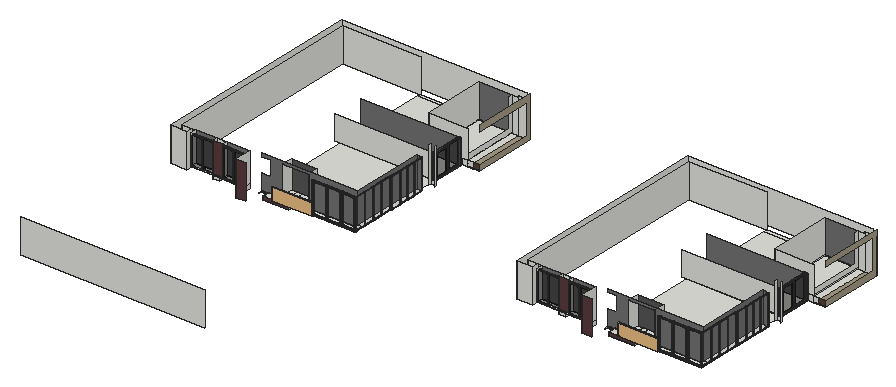
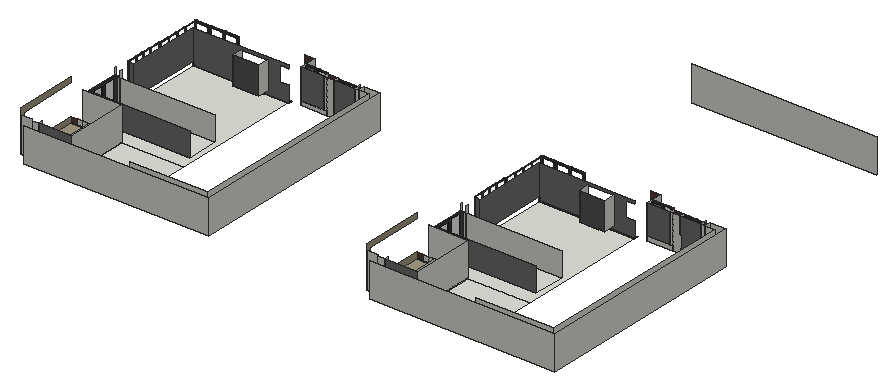
# SketchUp Ruby script. Lengths in inches.
U = 1.inch
M = Sketchup.active_model
def pt(a) = Geom::Point3d.new(a.map { |v| v * U })
def face(e, loops, mat)
  f = e.add_face(loops[0].map { |a| pt(a) })
  loops[1..].each { |l| e.add_face(l.map { |a| pt(a) }).erase! }
  f.material = f.back_material = mat if mat
  f
end
# faces: each face lists its corners as indices into pts; further lists are holes
def faces(e, pts, list, mat = nil) = list.each { |f| face(e, (f[0].is_a?(Array) ? f : [f]).map { |l| l.map { |i| pts[i] } }, mat) }
# xy, xz, yz: faces in a plane at the given z, y or x. An outline is a flat list of corners, or four numbers for a rectangle; further outlines are holes
def ring(l) = l.size == 4 ? [[l[0], l[1]], [l[2], l[1]], [l[2], l[3]], [l[0], l[3]]] : l.each_slice(2).to_a
def flat(e, list, mat, &to3) = list.each { |f| face(e, (f[0].is_a?(Array) ? f : [f]).map { |l| ring(l).map { |u, v| to3.(u, v) } }, mat) }
def xy(e, z, list, mat = nil) = flat(e, list, mat) { |x, y| [x, y, z] }
def xz(e, y, list, mat = nil) = flat(e, list, mat) { |x, z| [x, y, z] }
def yz(e, x, list, mat = nil) = flat(e, list, mat) { |y, z| [x, y, z] }
def lines(e, pts, list) = list.each { |a, b| e.add_line(pt(pts[a]), pt(pts[b])) }
# prism: a flat outline (further loops are holes) pulled along v
def prism(e, loops, v, mat = nil)
  f = face(e, loops, mat); d = Geom::Vector3d.new(v.map { |x| x * U })
  f.pushpull(f.normal.samedirection?(d) ? d.length : -d.length)
end
def box(e, o, s, mat = nil) = prism(e, [[o, [o[0] + s[0], o[1], o[2]], [o[0] + s[0], o[1] + s[1], o[2]], [o[0], o[1] + s[1], o[2]]]], [0, 0, s[2]], mat)
def at(x, y, z, deg = 0) = Geom::Transformation.translation(pt([x, y, z])) * Geom::Transformation.rotation(ORIGIN, Z_AXIS, deg.degrees)
def axes(o, x, y, z) = Geom::Transformation.new([*x, 0, *y, 0, *z, 0, *pt(o).to_a, 1])
def part(name) = M.definitions.add(name)
# library, detail: a bought-in or finely detailed component or shape, given as its bounding box
def library(name, o, s) = part(name).tap { |d| box(d.entities, o, s) }
def detail(e, o, s) = box(e.add_group.entities, o, s)
def put(e, d, t, mat = nil) = e.add_instance(d, t).tap { |i| i.material = mat if mat }
def group(e, t, mat = nil) = e.add_group.tap { |g| g.transformation = t; g.material = mat if mat }.entities
root = M.entities
M.materials.add("Glass_Tinted_Gray").color = [0, 0, 0]
M.materials["Glass_Tinted_Gray"].alpha = 0.125
M.materials.add("Glazing").color = [128, 128, 128]
M.materials["Glazing"].alpha = 0.05
M.materials.add("Powdercoating").color = [41, 44, 40]
M.materials.add("Wine2").color = [0, 0, 0]
M.materials["Wine2"].alpha = 0
M.materials.add("[0130_Gainsboro]").color = [39, 45, 50]
M.materials.add("[0135_DarkGray]").color = [81, 81, 81]
M.materials.add("[Color M05]").color = [114, 114, 114]
M.materials.add("[Color M06]").color = [86, 86, 86]
M.materials.add("[Concrete Tile]").color = [165, 155, 133]
M.materials.add("[Granite Brown]").color = [89, 59, 61]
M.materials.add("[Granite Brown]1").color = [89, 63, 50]
M.materials.add("[Mirror 02]").color = [229, 229, 229]
M.materials.add("[Terrazzo Light Blue]").color = [196, 214, 227]
c1 = library("Glass Railing",[0,0,0],[139.5,4.76,42])
c2 = part("Framed glazing panel")
xy(c2.entities,0,[[0,-0.98,43.07,0],[0,0,43.07,1.4]],"[0130_Gainsboro]")
xy(c2.entities,0.3,[[0.3,-1.43,42.77,-0.98]],"[0130_Gainsboro]")
xy(c2.entities,2.95,[[2.95,-1.43,40.12,-0.63],[2.95,-0.63,40.12,0],[2.95,0,40.12,0.64],[2.95,0.64,40.12,1.4]],"[0130_Gainsboro]")
xy(c2.entities,3.54,[[3.54,-0.63,39.53,0],[3.54,0,39.53,0.64]],"[0130_Gainsboro]")
xy(c2.entities,111.8125,[[3.54,-0.63,39.53,0],[3.54,0,39.53,0.64]],"[0130_Gainsboro]")
xy(c2.entities,112.4,[[2.95,-1.43,40.12,-0.63],[2.95,-0.63,40.12,0],[2.95,0,40.12,0.64],[2.95,0.64,40.12,1.4]],"[0130_Gainsboro]")
xy(c2.entities,115.05,[[0.3,-1.43,42.77,-0.98]],"[0130_Gainsboro]")
xy(c2.entities,115.35,[[0,-0.98,43.07,0],[0,0,43.07,1.4]],"[0130_Gainsboro]")
xz(c2.entities,-1.43,[[[0.3,0.3,42.77,115.05],[2.95,2.95,40.12,112.4]]],"[0130_Gainsboro]")
xz(c2.entities,-0.98,[[[0,0,43.07,115.35],[0.3,0.3,42.77,115.05]]],"[0130_Gainsboro]")
xz(c2.entities,-0.63,[[[2.95,2.95,40.12,112.4],[3.54,3.54,39.53,111.8125]]],"[0130_Gainsboro]")
xz(c2.entities,0,[[3.54,3.54,39.53,111.8125]],"Wine2")
xz(c2.entities,0,[[[0,0,43.07,115.35],[2.95,2.95,40.12,112.4]],[[2.95,2.95,40.12,112.4],[3.54,3.54,39.53,111.8125]]],"[0130_Gainsboro]")
xz(c2.entities,0.64,[[[2.95,2.95,40.12,112.4],[3.54,3.54,39.53,111.8125]]],"[0130_Gainsboro]")
xz(c2.entities,1.4,[[[0,0,43.07,115.35],[2.95,2.95,40.12,112.4]]],"[0130_Gainsboro]")
yz(c2.entities,0,[[-0.98,0,0,115.35],[0,0,1.4,115.35]],"[0130_Gainsboro]")
yz(c2.entities,0.3,[[-1.43,0.3,-0.98,115.05]],"[0130_Gainsboro]")
yz(c2.entities,2.95,[[-1.43,2.95,-0.63,112.4],[-0.63,2.95,0,112.4],[0,2.95,0.64,112.4],[0.64,2.95,1.4,112.4]],"[0130_Gainsboro]")
yz(c2.entities,3.54,[[-0.63,3.54,0,111.8125],[0,3.54,0.64,111.8125]],"[0130_Gainsboro]")
yz(c2.entities,39.53,[[-0.63,3.54,0,111.8125],[0,3.54,0.64,111.8125]],"[0130_Gainsboro]")
yz(c2.entities,40.12,[[-1.43,2.95,-0.63,112.4],[-0.63,2.95,0,112.4],[0,2.95,0.64,112.4],[0.64,2.95,1.4,112.4]],"[0130_Gainsboro]")
yz(c2.entities,42.77,[[-1.43,0.3,-0.98,115.05]],"[0130_Gainsboro]")
yz(c2.entities,43.07,[[-0.98,0,0,115.35],[0,0,1.4,115.35]],"[0130_Gainsboro]")
c3 = part("Glazed panel assembly")
put(c3.entities,c2,axes([90.57,1.43,0],[1.05148,0,0],[0,1,0],[0,0,1]))
put(c3.entities,c2,axes([0,1.43,0],[1.05148,0,0],[0,1,0],[0,0,1]))
put(c3.entities,c2,axes([45.29,1.43,0],[1.05148,0,0],[0,1,0],[0,0,1]))
c4 = part("PENTEK_RP Fineline 50S_Sliding_DoorCase_E1")
box(c4.entities,[0,0,0],[1.51,3.66,99.27],"[0135_DarkGray]")
c5 = part("PENTEK_RP Fineline 50S_SlidingDooe_Case_E2")
box(c5.entities,[0,0,0],[96.25,3.66,1.51],"[0135_DarkGray]")
c6 = part("pentek_RP Fineline 50S_SlidingDoor_Case")
put(c6.entities,c4,at(97.76,0,0))
put(c6.entities,c5,at(1.51,0,0))
put(c6.entities,c4,at(0,0,0))
put(c6.entities,c5,at(1.51,0,97.76))
c7 = part("PENTEK_RP Fineline 50S_SlidingDoor_GlazingBead_2")
box(c7.entities,[0,0,0],[0.56,0.59,94.39],"[0135_DarkGray]")
c8 = part("PENTEK_RP Fineline 50S_SlidingDoor_Glass")
box(c8.entities,[0,0,0],[46.58,0.16,94.39],"Glass_Tinted_Gray")
c9 = part("PENTEK_RP Fineline 50S_SlidingDoor_GlazingBead")
box(c9.entities,[0,0,0],[45.47,0.59,0.56],"[0135_DarkGray]")
c10 = part("PENTEK_RP Fineline 50S_SlidingDoor_Leaf_E1")
xy(c10.entities,0,[[0,0,0.93,1.97],[0.93,1.57,1.49,1.97]],"[0135_DarkGray]")
xy(c10.entities,96.25,[[0,0,0.93,0,0.93,1.57,1.49,1.57,1.49,1.97,0,1.97]],"[0135_DarkGray]")
xz(c10.entities,0,[[0,0,0.93,96.25]],"[0135_DarkGray]")
xz(c10.entities,1.57,[[0.93,0,1.49,95.32],[0.93,95.32,1.49,96.25]],"[0135_DarkGray]")
xz(c10.entities,1.97,[[0,0,1.49,96.25]],"[0135_DarkGray]")
yz(c10.entities,0,[[0,0,1.97,96.25]],"[0135_DarkGray]")
yz(c10.entities,0.93,[[0,0,1.57,0.93],[0,0.93,1.57,95.32],[0,95.32,1.57,96.25]],"[0135_DarkGray]")
yz(c10.entities,1.49,[[1.57,0,1.97,95.32],[1.57,95.32,1.97,96.25]],"[0135_DarkGray]")
c11 = part("PENTEK_RP Fineline 50S_SlidingDoor_Leaf_E2")
xy(c11.entities,0,[[0,0,0,1.57,0.56,1.57,0.56,1.97,46.02,1.97,46.02,1.57,46.58,1.57,46.58,0]],"[0135_DarkGray]")
xy(c11.entities,0.93,[[0,0,46.58,1.57]],"[0135_DarkGray]")
xy(c11.entities,1.49,[[0.56,1.57,46.02,1.97]],"[0135_DarkGray]")
xz(c11.entities,0,[[0,0,46.58,0.93]],"[0135_DarkGray]")
xz(c11.entities,1.57,[[0,0,0.56,0.93],[46.02,0,46.58,0.93],[0.56,0.93,46.02,1.49]],"[0135_DarkGray]")
xz(c11.entities,1.97,[[0.56,0,46.02,1.49]],"[0135_DarkGray]")
yz(c11.entities,0,[[0,0,1.57,0.93]],"[0135_DarkGray]")
yz(c11.entities,0.56,[[1.57,0,1.97,0.93],[1.57,0.93,1.97,1.49]],"[0135_DarkGray]")
yz(c11.entities,46.02,[[1.57,0,1.97,0.93],[1.57,0.93,1.97,1.49]],"[0135_DarkGray]")
yz(c11.entities,46.58,[[0,0,1.57,0.93]],"[0135_DarkGray]")
c12 = part("PENTEK_RP Fineline S_SlidingDoor_Leaf1")
put(c12.entities,c7,at(0.93,0,0.93))
put(c12.entities,c7,at(46.96,0,0.93))
put(c12.entities,c8,at(1.49,1.42,0.93))
put(c12.entities,c9,at(1.49,0,0.93))
put(c12.entities,c8,at(1.49,0.59,0.93),"[Terrazzo Light Blue]")
put(c12.entities,c10,at(0,0,0))
put(c12.entities,c10,axes([48.44,0,0],[-1,0,0],[0,1,0],[0,0,1]))
put(c12.entities,c11,axes([0.93,0,96.25],[1,0,0],[0,1,0],[0,0,-1]))
put(c12.entities,c11,at(0.93,0,0))
put(c12.entities,c9,at(1.49,0,94.77))
c13 = part("PENTEK_RP Fineline 50S_SlidingDoor_Leaf2")
put(c13.entities,c8,at(1.49,1.42,0.93))
put(c13.entities,c9,at(1.49,0,94.77))
put(c13.entities,c7,at(46.96,0,0.93))
put(c13.entities,c8,at(1.49,0.59,0.93),"[Mirror 02]")
put(c13.entities,c7,at(0.93,0,0.93))
put(c13.entities,c10,at(0,0,0))
put(c13.entities,c10,axes([48.44,0,0],[-1,0,0],[0,1,0],[0,0,1]))
put(c13.entities,c9,at(1.49,0,0.93))
put(c13.entities,c11,axes([0.93,0,96.25],[1,0,0],[0,1,0],[0,0,-1]))
put(c13.entities,c11,at(0.93,0,0))
c14 = part("PENTEK - Slimmest Steel Sliding Door / Window\#1")
put(c14.entities,c6,at(0,-1.88,-0.09))
put(c14.entities,c12,at(1.51,-2.27,1.42))
put(c14.entities,c13,at(49.32,-0.3,1.42))
c15 = part("Group\#15")
xy(c15.entities,0,[[0,-55.94,0.71,45.94]])
xy(c15.entities,0.2,[[0,-55.94,0.47,45.94],[0.47,45.94,0.71,46.42]])
xy(c15.entities,2.36,[[0.47,-55.94,0.71,46.42]])
xz(c15.entities,-55.94,[[0,0,0.71,0,0.71,2.36,0.47,2.36,0.47,0.2,0,0.2]])
xz(c15.entities,45.94,[[0,0,0.71,0.2]])
xz(c15.entities,46.42,[[0.47,0.2,0.71,2.36]])
yz(c15.entities,0,[[-55.94,0,45.94,0.2]])
yz(c15.entities,0.47,[[-55.94,0.2,46.42,2.36]])
yz(c15.entities,0.71,[[-55.94,0,45.94,0,45.94,0.2,46.42,0.2,46.42,2.36,-55.94,2.36]])
c16 = part("Group\#7")
xy(c16.entities,0,[[0,-59.09,0.71,45.94]])
xy(c16.entities,0.2,[[0,-59.09,0.47,45.94],[0.47,45.94,0.71,46.42]])
xy(c16.entities,2.36,[[0.47,-59.09,0.71,46.42]])
xz(c16.entities,-59.09,[[0,0,0.71,0,0.71,2.36,0.47,2.36,0.47,0.2,0,0.2]])
xz(c16.entities,45.94,[[0,0,0.71,0.2]])
xz(c16.entities,46.42,[[0.47,0.2,0.71,2.36]])
yz(c16.entities,0,[[-59.09,0,45.94,0.2]])
yz(c16.entities,0.47,[[-59.09,0.2,46.42,2.36]])
yz(c16.entities,0.71,[[-59.09,0,45.94,0,45.94,0.2,46.42,0.2,46.42,2.36,-59.09,2.36]])
c17 = part("Group\#16")
prism(c17.entities,[[[0.47,-56.18,0.2],[0,-56.18,0.2],[0,-56.18,0],[0.71,-56.18,0],[0.71,-56.18,2.36],[0.47,-56.18,2.36]]],[0,28.68,0])
c18 = part("Group\#10")
box(c18.entities,[-0.73,0,0],[27.99,0.55,102.05])
c19 = part("Group\#18")
xy(c19.entities,0,[[0.47,-56.18,0.47,-55.47,0,-55.47,0,-28.21,1.18,-28.21,1.18,-56.18]])
xy(c19.entities,0.2,[[0.71,-56.18,1.18,-28.21],[0,-55.47,0.47,-28.21],[0.47,-28.21,0.71,-27.74]])
xy(c19.entities,2.36,[[0.47,-56.18,0.71,-27.74]])
xz(c19.entities,-56.18,[[0.47,0,1.18,0,1.18,0.2,0.71,0.2,0.71,2.36,0.47,2.36]])
xz(c19.entities,-55.47,[[0,0,0.47,0.2]])
xz(c19.entities,-28.21,[[0,0,1.18,0.2]])
xz(c19.entities,-27.74,[[0.47,0.2,0.71,2.36]])
yz(c19.entities,0,[[-55.47,0,-28.21,0.2]])
yz(c19.entities,0.47,[[-56.18,0,-55.47,0.2],[-56.18,0.2,-27.74,2.36]])
yz(c19.entities,0.71,[[-56.18,0.2,-27.74,2.36]])
yz(c19.entities,1.18,[[-56.18,0,-28.21,0.2]])
c20 = part("Group\#34")
xy(c20.entities,0,[[-20.45,0,7.76,1.22]])
xy(c20.entities,0.06,[[-20.39,0.06,7.7,1.22]])
xy(c20.entities,0.47,[[-19.98,0,7.28,0.06]])
xy(c20.entities,101.89,[[-19.98,0,7.28,0.06]])
xy(c20.entities,102.3,[[-20.39,0.06,7.7,1.22]])
xy(c20.entities,102.36,[[-20.45,0,7.76,1.22]])
xz(c20.entities,0,[[[-20.45,0,7.76,102.36],[-19.98,0.47,7.28,101.89]]])
xz(c20.entities,0.06,[[[-20.39,0.06,7.7,102.3],[-19.98,0.47,7.28,101.89]]])
xz(c20.entities,1.22,[[[-20.45,0,7.76,102.36],[-20.39,0.06,7.7,102.3]]])
yz(c20.entities,-20.45,[[0,0,1.22,102.36]])
yz(c20.entities,-20.39,[[0.06,0.06,1.22,102.3]])
yz(c20.entities,-19.98,[[0,0.47,0.06,101.89]])
yz(c20.entities,7.28,[[0,0.47,0.06,101.89]])
yz(c20.entities,7.7,[[0.06,0.06,1.22,102.3]])
yz(c20.entities,7.76,[[0,0,1.22,102.36]])
c21 = part("Group\#6")
put(c21.entities,c15,axes([27.97,0,7.875],[1,0,0],[0,0,-1],[0,1,0]),"Powdercoating")
put(c21.entities,c16,axes([0.71,0,6.8],[-1,0,0],[0,0,-0.97687],[0,1,0]),"Powdercoating")
put(c21.entities,c17,axes([-27.5,0,-38.07],[0,0,-1],[-1,0,0],[0,1,0]),"Powdercoating")
put(c21.entities,c18,at(1.12,0.35,-38.39),"Glazing")
put(c21.entities,c19,axes([-27.5,0,63.35],[0,0,1],[-1,0,0],[0,1,0]),"Powdercoating")
put(c21.entities,c20,at(20.6875,1.0625,-38.54),"Powdercoating")
c22 = part("Sliding door assembly")
put(c22.entities,c21,at(-1.18,4.5,38.86))
g1 = group(c22.entities,at(84.74,4.5,38.86))
put(g1,c15,axes([-27.97,0,7.875],[-1,0,0],[0,0,-1],[0,1,0]),"Powdercoating")
put(g1,c16,axes([-0.71,0,6.8],[1,0,0],[0,0,-0.97687],[0,1,0]),"Powdercoating")
put(g1,c17,axes([27.5,0,-38.07],[0,0,-1],[1,0,0],[0,1,0]),"Powdercoating")
put(g1,c18,axes([-1.12,0.35,-38.39],[-1,0,0],[0,1,0],[0,0,1]),"Glazing")
put(g1,c19,axes([27.5,0,63.35],[0,0,1],[1,0,0],[0,1,0]),"Powdercoating")
put(g1,c20,axes([-20.6875,1.0625,-38.54],[-1,0,0],[0,1,0],[0,0,1]),"Powdercoating")
g2 = group(c22.entities,at(56.0625,4.5,38.86))
put(g2,c15,axes([-27.97,0,7.875],[-1,0,0],[0,0,-1],[0,1,0]),"Powdercoating")
put(g2,c17,axes([27.5,0,-38.07],[0,0,-1],[1,0,0],[0,1,0]),"Powdercoating")
put(g2,c18,axes([-1.12,0.35,-38.39],[-1,0,0],[0,1,0],[0,0,1]),"Glazing")
put(g2,c19,axes([27.5,0,63.35],[0,0,1],[1,0,0],[0,1,0]),"Powdercoating")
put(g2,c20,axes([-20.6875,1.0625,-38.54],[-1,0,0],[0,1,0],[0,0,1]),"Powdercoating")
g3 = group(g2,at(-0.71,0,6.8),"Powdercoating")
xy(g3,-45.34,[[0.47,0.2,0.71,2.36]])
xy(g3,-44.88,[[0,0,0.71,0.2]])
xy(g3,57.73,[[0,0,0.71,0,0.71,2.36,0.47,2.36,0.47,0.2,0,0.2]])
xz(g3,0,[[0,-44.88,0.71,57.73]])
xz(g3,0.2,[[0.47,-45.34,0.71,-44.88],[0,-44.88,0.47,57.73]])
xz(g3,2.36,[[0.47,-45.34,0.71,57.73]])
yz(g3,0,[[0,-44.88,0.2,57.73]])
yz(g3,0.47,[[0.2,-45.34,2.36,57.73]])
yz(g3,0.71,[[0.2,-45.34,2.36,-45.34,2.36,57.73,0,57.73,0,-44.88,0.2,-44.88]])
put(c22.entities,c21,axes([-33.94,4.5,38.86],[1.14218,0,0],[0,1,0],[0,0,1]))
c23 = part("sliding door")
put(c23.entities,c22,at(0,-4.5,-0.08))
xy(root,1518,[[589.7,3214.625,679.51,3237.625],[1807.88,3214.625,1897.7,3237.625],[557.88,3237.625,558.625,3249.875],[679.51,3237.625,890.875,3243.6875],[1776.07,3237.625,1776.8125,3249.875],
  [1897.7,3237.625,2109.0625,3243.6875],[558.625,3243.6875,679.51,3249.875],[679.51,3243.6875,890.875,3249.875],[1776.8125,3243.6875,1897.7,3249.875],[1897.7,3243.6875,2109.0625,3249.875],
  [558.625,3249.875,890.875,3710.5625],[1776.8125,3249.875,2109.0625,3710.5625],[558.625,3710.5625,774.6875,3933.57],[774.6875,3710.5625,890.875,3933.57],[890.875,3710.5625,913.875,3933.57],
  [1776.8125,3710.5625,1992.875,3933.57],[1992.875,3710.5625,2109.0625,3933.57],[2109.0625,3710.5625,2132.0625,3933.57],[558.625,3933.57,890.875,3946.0625],[1776.8125,3933.57,2109.0625,3946.0625]])
xy(root,1518,[[913.875,3710.5625,954.6875,3933.57],[2132.0625,3710.5625,2172.875,3933.57]],"[Concrete Tile]")
xy(root,1518,[[557.4,3237.625,557.88,3249.875],[1775.59,3237.625,1776.07,3249.875]],"[Granite Brown]")
xy(root,1519.75,[[774.6875,3710.5625,890.875,3933.57],[1992.875,3710.5625,2109.0625,3933.57]])
xy(root,1519.8125,[[558.625,3243.6875,890.875,3249.875],[1776.8125,3243.6875,2109.0625,3249.875]])
xy(root,1530.6875,[[589.7,3214.625,679.51,3237.625],[679.51,3214.625,913.875,3214.625,913.875,3249.875,890.875,3249.875,890.875,3237.625,679.51,3237.625],[1807.88,3214.625,1897.7,3237.625],[1897.7,3214.625,2132.0625,3214.625,2132.0625,3249.875,2109.0625,3249.875,2109.0625,3237.625,1897.7,3237.625],[894.3125,3249.875,913.875,3508.84],
  [2112.5,3249.875,2132.0625,3508.84]])
xy(root,1531.38,[[652.3,3249.875,668.6,3288.0625],[668.6,3249.875,670.29,3288.0625],[670.29,3249.875,721.4,3288.0625],[1870.49,3249.875,1886.79,3288.0625],[1886.79,3249.875,1888.48,3288.0625],
  [1888.48,3249.875,1939.59,3288.0625]])
xy(root,1531.7,[[631.46,3249.875,652.3,3288.0625],[1849.65,3249.875,1870.49,3288.0625]])
xy(root,1533.4375,[[333.68,3214.625,523.04,3214.625,523.04,3237.625,442.15,3237.625,442.15,3221.25,406.21,3221.25,406.21,3237.625,333.68,3237.625],[1551.87,3214.625,1741.23,3214.625,1741.23,3237.625,1660.33,3237.625,1660.33,3221.25,1624.4,3221.25,1624.4,3237.625,1551.87,3237.625],[431.33,3221.25,442.15,3237.625],[1649.52,3221.25,1660.33,3237.625]])
xy(root,1535.36,[[558.625,3570.7,913.875,3681.01],[1776.8125,3570.7,2132.0625,3681.01]])
xz(root,2554.375,[[262.875,1518,913.875,1638]])
xz(root,3177.9375,[[523.04,1518,557.88,1638],[1741.23,1518,1776.07,1638]],"[Granite Brown]")
xz(root,3214.625,[[262.875,1518,319.53,1638],[1481.0625,1518,1537.72,1638]])
xz(root,3214.625,[[589.7,1518,679.51,1530.6875],[1807.88,1518,1897.7,1530.6875]],"[Granite Brown]")
xz(root,3221.25,[[406.21,1518,406.21,1533.4375,406.29,1533.4375],[406.21,1518,431.33,1518,431.33,1533.4375,406.29,1533.4375],[1624.4,1518,1624.4,1533.4375,1624.48,1533.4375],[1624.4,1518,1649.52,1518,1649.52,1533.4375,1624.48,1533.4375]])
xz(root,3221.25,[[406.29,1533.4375,442.15,1533.4375,442.15,1638,406.8125,1638],[1624.48,1533.4375,1660.33,1533.4375,1660.33,1638,1625,1638]],"[Granite Brown]")
xz(root,3237.625,[[285.875,1518,319.53,1638],[319.53,1518,406.21,1518,406.21,1533.4375,333.68,1533.4375,333.68,1638,319.53,1638],[406.21,1518,406.8125,1638,431.33,1638,431.33,1518],[431.33,1518,523.04,1533.4375],[589.7,1518,679.51,1530.6875],
  [679.51,1518,890.875,1530.6875],[1504.0625,1518,1537.72,1638],[1537.72,1518,1624.4,1518,1624.4,1533.4375,1551.87,1533.4375,1551.87,1638,1537.72,1638],[1624.4,1518,1625,1638,1649.52,1638,1649.52,1518],[1649.52,1518,1741.23,1533.4375],
  [1807.88,1518,1897.7,1530.6875],[1897.7,1518,2109.0625,1530.6875],[431.33,1533.4375,442.15,1638],[1649.52,1533.4375,1660.33,1638]])
xz(root,3237.625,[[406.21,1518,406.8125,1638,333.68,1638,333.68,1533.4375,406.21,1533.4375],[1624.4,1518,1625,1638,1551.87,1638,1551.87,1533.4375,1624.4,1533.4375],[442.15,1533.4375,523.04,1638],[1660.33,1533.4375,1741.23,1638]],"[Color M05]")
xz(root,3243.6875,[[558.625,1518,890.875,1519.8125],[1776.8125,1518,2109.0625,1519.8125]])
xz(root,3249.875,[[558.625,1518,890.875,1519.8125],[890.875,1518,894.3125,1530.6875],[1776.8125,1518,2109.0625,1519.8125],[2109.0625,1518,2112.5,1530.6875]])
xz(root,3249.875,[[[557.88,1518,558.625,1518,558.625,1519.8125,890.875,1519.8125,890.875,1530.6875,894.3125,1530.6875,894.3125,1638,557.88,1638,557.88,1627.45,588.66,1627.45,588.66,1575.17,557.88,1575.17],[652.3,1531.38,652.3,1531.7,631.46,1531.7,631.46,1629.51,721.4,1629.51,721.4,1531.38]],[[1776.07,1518,1776.8125,1518,1776.8125,1519.8125,2109.0625,1519.8125,2109.0625,1530.6875,2112.5,1530.6875,2112.5,1638,1776.07,1638,1776.07,1627.45,1806.84,1627.45,1806.84,1575.17,1776.07,1575.17],[1870.49,1531.38,1870.49,1531.7,1849.65,1531.7,1849.65,1629.51,1939.59,1629.51,1939.59,1531.38]]],"[Color M05]")
xz(root,3288.0625,[[652.3,1531.38,721.4,1531.38,721.4,1629.51,631.46,1629.51,631.46,1531.7,652.3,1531.7],[1870.49,1531.38,1939.59,1531.38,1939.59,1629.51,1849.65,1629.51,1849.65,1531.7,1870.49,1531.7]],"[Color M06]")
xz(root,3508.84,[[894.3125,1530.6875,913.875,1638],[2112.5,1530.6875,2132.0625,1638]],"[Color M05]")
xz(root,3570.7,[[894.3125,1518,913.875,1535.36],[2112.5,1518,2132.0625,1535.36],[558.625,1535.36,894.3125,1621.04],[894.3125,1535.36,913.875,1621.04],[1776.8125,1535.36,2112.5,1621.04],
  [2112.5,1535.36,2132.0625,1621.04]])
xz(root,3681.01,[[558.625,1535.36,913.875,1621.04],[1776.8125,1535.36,2132.0625,1621.04]],"[Color M05]")
xz(root,3710.5625,[[774.6875,1518,890.875,1519.75],[890.875,1518,913.875,1538.8125],[913.875,1518,930.75,1519.75],[930.75,1518,954.6875,1519.75],[1992.875,1518,2109.0625,1519.75],
  [2109.0625,1518,2132.0625,1538.8125],[2132.0625,1518,2148.9375,1519.75],[2148.9375,1518,2172.875,1519.75],[774.6875,1519.75,774.6875,1638,913.875,1638,913.875,1538.8125,890.875,1538.8125,890.875,1519.75],[913.875,1519.75,930.75,1538.8125],
  [1992.875,1519.75,1992.875,1638,2132.0625,1638,2132.0625,1538.8125,2109.0625,1538.8125,2109.0625,1519.75],[2132.0625,1519.75,2148.9375,1538.8125]])
xz(root,3710.5625,[[930.75,1519.75,954.6875,1538.8125],[2148.9375,1519.75,2172.875,1538.8125]],"[Granite Brown]1")
xz(root,3933.57,[[774.6875,1518,890.875,1519.75],[890.875,1518,913.875,1638],[913.875,1518,954.6875,1643.375],[1992.875,1518,2109.0625,1519.75],[2109.0625,1518,2132.0625,1638],
  [2132.0625,1518,2172.875,1643.375]])
xz(root,3933.57,[[774.6875,1519.75,890.875,1638],[1992.875,1519.75,2109.0625,1638]],"[Color M05]")
xz(root,3946.0625,[[285.875,1518,558.625,1638],[1504.0625,1518,1776.8125,1638]])
xz(root,3969.0625,[[262.875,1518,913.875,1638],[1481.0625,1518,2132.0625,1638]])
yz(root,262.875,[[3214.625,1518,3969.0625,1638]])
yz(root,285.875,[[3237.625,1518,3946.0625,1638]])
yz(root,319.53,[[3214.625,1518,3237.625,1638]])
yz(root,333.68,[[3214.625,1533.4375,3237.625,1638]])
yz(root,406.21,[[3221.25,1518,3237.625,1533.4375]])
yz(root,431.33,[[3221.25,1518,3237.625,1533.4375]])
yz(root,442.15,[[3221.25,1533.4375,3237.625,1638]])
yz(root,523.04,[[3177.9375,1518,3214.625,1533.4375],[3214.625,1518,3237.625,1533.4375],[3177.9375,1533.4375,3237.625,1638]])
yz(root,558.625,[[3237.625,1518,3243.6875,1519.8125],[3243.6875,1518,3249.875,1519.8125]])
yz(root,589.7,[[3214.625,1518,3237.625,1530.6875]],"[Granite Brown]")
yz(root,631.46,[[3249.875,1531.7,3288.0625,1629.51]])
yz(root,652.3,[[3249.875,1531.38,3288.0625,1531.7]])
yz(root,679.51,[[3214.625,1518,3237.625,1530.6875]])
yz(root,721.4,[[3249.875,1531.38,3288.0625,1629.51]])
yz(root,774.6875,[[3710.5625,1518,3933.57,1519.75],[3710.5625,1519.75,3933.57,1638]])
yz(root,890.875,[[3237.625,1518,3243.6875,1530.6875],[3243.6875,1518,3249.875,1519.8125],[3710.5625,1518,3933.57,1519.75],[3710.5625,1519.75,3710.5625,1538.8125,3919.9,1538.8125,3919.9,1638,3933.57,1638,3933.57,1519.75],[3243.6875,1519.8125,3249.875,1530.6875]])
yz(root,894.3125,[[3563.51,1518,3570.7,1644]])
yz(root,894.3125,[[3249.875,1530.6875,3508.84,1638]],"[Color M05]")
yz(root,913.875,[[3563.51,1518,3570.7,1644]])
yz(root,954.6875,[[3710.5625,1518,3933.57,1518,3933.57,1663.0625,3710.5625,1663.0625,3710.5625,1643.375,3919.9,1643.375,3919.9,1538.8125,3710.5625,1538.8125]],"[Concrete Tile]")
yz(root,1481.0625,[[3214.625,1518,3969.0625,1638]])
yz(root,1504.0625,[[3237.625,1518,3946.0625,1638]])
yz(root,1537.72,[[3214.625,1518,3237.625,1638]])
yz(root,1551.87,[[3214.625,1533.4375,3237.625,1638]])
yz(root,1624.4,[[3221.25,1518,3237.625,1533.4375]])
yz(root,1649.52,[[3221.25,1518,3237.625,1533.4375]])
yz(root,1660.33,[[3221.25,1533.4375,3237.625,1638]])
yz(root,1741.23,[[3177.9375,1518,3214.625,1533.4375],[3214.625,1518,3237.625,1533.4375],[3177.9375,1533.4375,3237.625,1638]])
yz(root,1776.8125,[[3237.625,1518,3243.6875,1519.8125],[3243.6875,1518,3249.875,1519.8125]])
yz(root,1807.88,[[3214.625,1518,3237.625,1530.6875]],"[Granite Brown]")
yz(root,1849.65,[[3249.875,1531.7,3288.0625,1629.51]])
yz(root,1870.49,[[3249.875,1531.38,3288.0625,1531.7]])
yz(root,1897.7,[[3214.625,1518,3237.625,1530.6875]])
yz(root,1939.59,[[3249.875,1531.38,3288.0625,1629.51]])
yz(root,1992.875,[[3710.5625,1518,3933.57,1519.75],[3710.5625,1519.75,3933.57,1638]])
yz(root,2109.0625,[[3237.625,1518,3243.6875,1530.6875],[3243.6875,1518,3249.875,1519.8125],[3710.5625,1518,3933.57,1519.75],[3710.5625,1519.75,3710.5625,1538.8125,3919.9,1538.8125,3919.9,1638,3933.57,1638,3933.57,1519.75],[3243.6875,1519.8125,3249.875,1530.6875]])
yz(root,2112.5,[[3563.51,1518,3570.7,1644]])
yz(root,2112.5,[[3249.875,1530.6875,3508.84,1638]],"[Color M05]")
yz(root,2132.0625,[[3563.51,1518,3570.7,1644]])
yz(root,2172.875,[[3710.5625,1518,3933.57,1518,3933.57,1663.0625,3710.5625,1663.0625,3710.5625,1643.375,3919.9,1643.375,3919.9,1538.8125,3710.5625,1538.8125]],"[Concrete Tile]")
p = [[406.21,3237.625,1518],[406.21,3221.25,1518],[406.29,3221.25,1533.4375],[406.8125,3221.25,1638],[406.8125,3237.625,1638],[1624.4,3237.625,1518],
  [1624.4,3221.25,1518],[1624.48,3221.25,1533.4375],[1625,3221.25,1638],[1625,3237.625,1638]]
faces(root,p,[[0,1,2,3,4],[5,6,7,8,9]])
put(root,c1,at(1840.53,3212.87,1527.4))
put(root,c1,at(622.34,3212.87,1527.4))
put(root,c3,axes([1979.67,3214.625,1530.6875],[1.12166,0,0],[0,1,0],[0,0,0.95]))
put(root,c3,axes([761.48,3214.625,1530.6875],[1.12166,0,0],[0,1,0],[0,0,0.95]))
put(root,c14,axes([1664.65,3216.5,1533.53],[0.7714,0,0],[0,1,0],[0,0,1.054]))
put(root,c14,axes([446.46,3216.5,1533.53],[0.7714,0,0],[0,1,0],[0,0,1.054]))
put(root,c14,axes([1550.21,3221.55,1530.375],[0.7714,0,0],[0,1,0],[0,0,1.054]))
put(root,c14,axes([332.02,3221.55,1530.375],[0.7714,0,0],[0,1,0],[0,0,1.054]))
put(root,c23,axes([2132.0625,3259.26,1530.6875],[0,1.302,0],[-1,0,0],[0,0,1.03877]))
put(root,c23,axes([913.875,3259.26,1530.6875],[0,1.302,0],[-1,0,0],[0,0,1.03877]))
put(root,c23,axes([2134.42,3410.41,1531.32],[0,1.13453,0],[-1,0,0],[0,0,1.03262]))
put(root,c23,axes([916.24,3410.41,1531.32],[0,1.13453,0],[-1,0,0],[0,0,1.03262]))
put(root,c14,axes([2126.35,3569.65,1535.4375],[0,1.12181,0],[-2.51374,0,0],[0,0,0.87918]))
put(root,c14,axes([908.17,3569.65,1535.4375],[0,1.12181,0],[-2.51374,0,0],[0,0,0.87918]))
